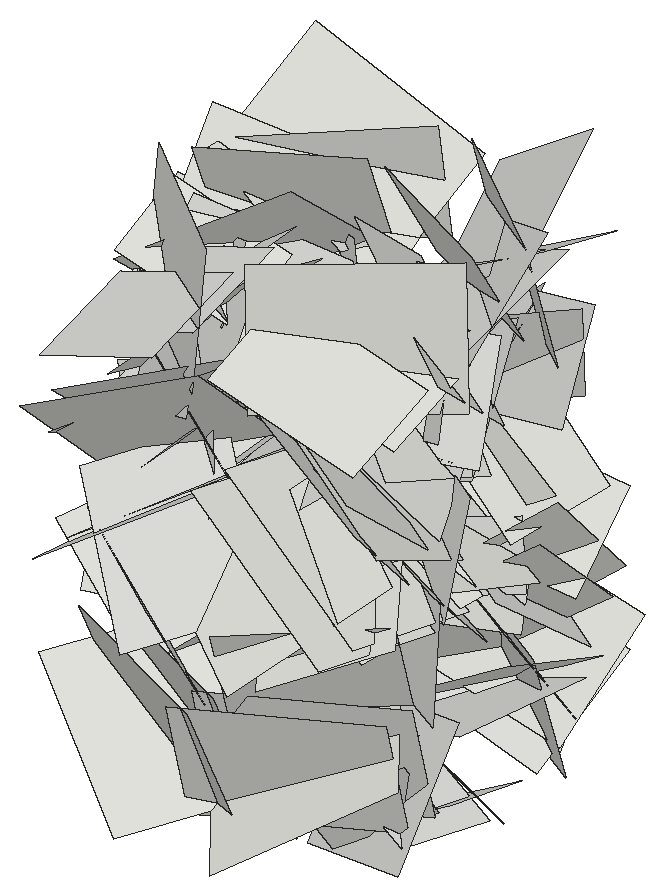
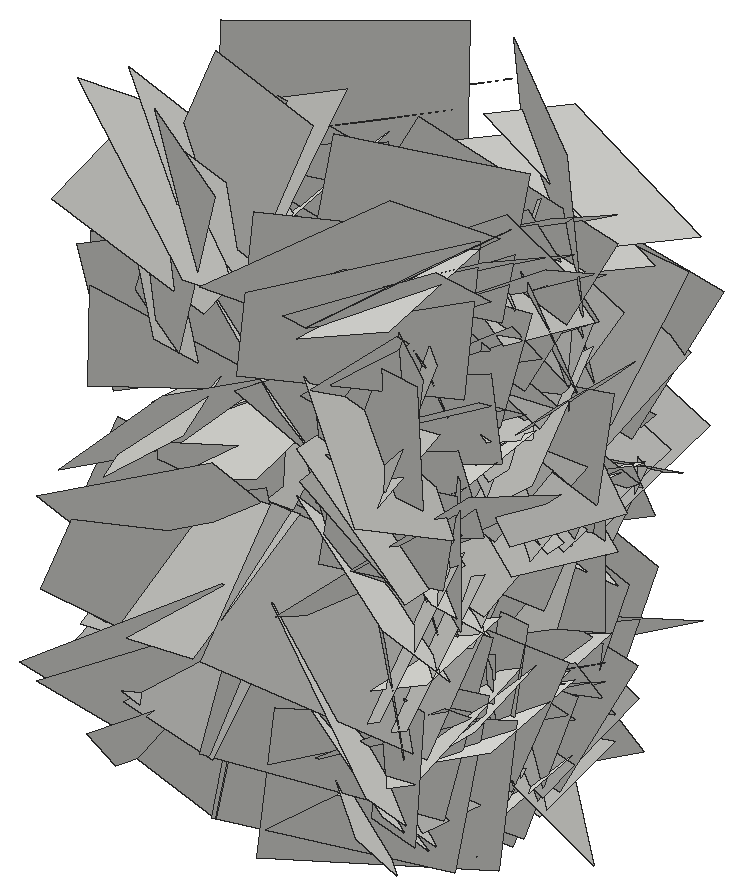
# SketchUp Ruby script. Lengths in inches.
U = 1.inch
M = Sketchup.active_model
def pt(a) = Geom::Point3d.new(a.map { |v| v * U })
def face(e, loops, mat)
  f = e.add_face(loops[0].map { |a| pt(a) })
  loops[1..].each { |l| e.add_face(l.map { |a| pt(a) }).erase! }
  f.material = f.back_material = mat if mat
  f
end
# faces: each face lists its corners as indices into pts; further lists are holes
def faces(e, pts, list, mat = nil) = list.each { |f| face(e, (f[0].is_a?(Array) ? f : [f]).map { |l| l.map { |i| pts[i] } }, mat) }
# xy, xz, yz: faces in a plane at the given z, y or x. An outline is a flat list of corners, or four numbers for a rectangle; further outlines are holes
def ring(l) = l.size == 4 ? [[l[0], l[1]], [l[2], l[1]], [l[2], l[3]], [l[0], l[3]]] : l.each_slice(2).to_a
def flat(e, list, mat, &to3) = list.each { |f| face(e, (f[0].is_a?(Array) ? f : [f]).map { |l| ring(l).map { |u, v| to3.(u, v) } }, mat) }
def xy(e, z, list, mat = nil) = flat(e, list, mat) { |x, y| [x, y, z] }
def xz(e, y, list, mat = nil) = flat(e, list, mat) { |x, z| [x, y, z] }
def yz(e, x, list, mat = nil) = flat(e, list, mat) { |y, z| [x, y, z] }
def lines(e, pts, list) = list.each { |a, b| e.add_line(pt(pts[a]), pt(pts[b])) }
# prism: a flat outline (further loops are holes) pulled along v
def prism(e, loops, v, mat = nil)
  f = face(e, loops, mat); d = Geom::Vector3d.new(v.map { |x| x * U })
  f.pushpull(f.normal.samedirection?(d) ? d.length : -d.length)
end
def box(e, o, s, mat = nil) = prism(e, [[o, [o[0] + s[0], o[1], o[2]], [o[0] + s[0], o[1] + s[1], o[2]], [o[0], o[1] + s[1], o[2]]]], [0, 0, s[2]], mat)
def at(x, y, z, deg = 0) = Geom::Transformation.translation(pt([x, y, z])) * Geom::Transformation.rotation(ORIGIN, Z_AXIS, deg.degrees)
def axes(o, x, y, z) = Geom::Transformation.new([*x, 0, *y, 0, *z, 0, *pt(o).to_a, 1])
def part(name) = M.definitions.add(name)
# library, detail: a bought-in or finely detailed component or shape, given as its bounding box
def library(name, o, s) = part(name).tap { |d| box(d.entities, o, s) }
def detail(e, o, s) = box(e.add_group.entities, o, s)
def put(e, d, t, mat = nil) = e.add_instance(d, t).tap { |i| i.material = mat if mat }
def group(e, t, mat = nil) = e.add_group.tap { |g| g.transformation = t; g.material = mat if mat }.entities
root = M.entities
c1 = part("Component\#6")
p = [[0.01,0,0],[0,3.24,4.54],[4.32,3.24,4.54],[4.33,0,0]]
faces(c1.entities,p,[[0,1,2,3]])
put(root,c1,axes([24.34,132.67,11.61],[-0.16439,-1.14375,-0.17253],[-0.24163,-0.14044,1.13591],[1.20204,-0.18465,0.20475]))
put(root,c1,axes([28.31,132.67,11.61],[0.16439,-1.14375,-0.17253],[0.24163,-0.14044,1.13591],[-1.20204,-0.18465,0.20475]))
put(root,c1,axes([24.34,126.24,11.02],[0.17433,0.41563,0.4957],[0.04437,0.50356,-0.43611],[0.68427,-0.13854,-0.09801]))
put(root,c1,axes([28.31,133.51,8.98],[0.15319,0.47062,-0.90401],[0.09722,-0.91536,-0.46187],[-1.07594,-0.0157,-0.17044]))
put(root,c1,axes([24.34,136.01,11.51],[0.06598,-0.27091,0.62957],[0.16839,0.62065,0.25136],[0.70672,-0.12259,-0.11867]))
put(root,c1,axes([24.34,130.2,1.79],[-0.1042,-0.77086,0.73803],[-0.17604,0.74317,0.75412],[1.11745,0.04519,0.18762]))
put(root,c1,axes([24.34,137.27,19.36],[-0.1763,0.15017,-0.9005],[0.15684,-0.89878,-0.17721],[0.95491,0.17535,-0.13715]))
put(root,c1,axes([28.31,136.42,13.64],[-0.14309,-0.55174,0.41683],[0.03038,0.41987,0.56505],[-0.73236,0.12522,-0.058]))
put(root,c1,axes([28.31,135.65,2.32],[0.1935,-1.06071,0.09437],[0.13048,0.11613,1.0671],[-1.12123,-0.16954,0.14047]))
put(root,c1,axes([24.34,132.96,18.89],[-0.10145,-0.91774,-0.17179],[0.02227,-0.17476,0.92192],[0.98945,-0.09016,-0.03837]))
put(root,c1,axes([24.34,133.07,14.74],[-0.12706,0.28525,0.91315],[0.02767,0.92092,-0.28425],[1.01369,0.01061,0.12222]))
put(root,c1,axes([24.34,135.14,15.06],[-0.15738,0.18416,-1.10832],[-0.16264,-1.1108,-0.16402],[1.17977,-0.12857,-0.17046]))
put(root,c1,axes([28.31,130.01,4.69],[-0.05447,0.12092,0.77662],[0.06993,0.77619,-0.11649],[-0.83019,0.05744,-0.06077]))
put(root,c1,axes([24.34,131.35,15.19],[0.02447,0.82058,-0.14823],[0.01236,-0.14859,-0.82075],[0.8838,-0.02064,0.01558]))
put(root,c1,axes([24.34,133.58,20.74],[-0.06025,0.71815,0.57437],[-0.00066,0.57544,-0.71955],[0.97476,0.04478,0.03501]))
put(root,c1,axes([24.34,133.14,16.06],[-0.03738,-0.31853,0.81486],[0.04959,0.81367,0.32009],[0.92608,-0.05642,0.01575]))
put(root,c1,axes([28.31,137.37,4.77],[0.01509,-0.67708,-0.46908],[0.05072,-0.46768,0.67651],[-0.87164,-0.03894,0.03124]))
put(root,c1,axes([24.34,128.53,16.93],[-0.30517,1.08519,-0.55956],[-0.1011,-0.59314,-1.10124],[1.29027,0.21019,-0.21864]))
put(root,c1,axes([24.34,127.92,4.7],[0.092,0.70183,0.2556],[0.07294,0.24871,-0.70628],[0.78837,-0.10491,0.03552]))
put(root,c1,axes([24.34,125.93,11.7],[0.16945,0.67455,-0.05214],[0.09647,-0.07453,-0.68517],[0.71064,-0.15073,0.10544]))
put(root,c1,axes([28.31,136.82,15.87],[0.16772,-0.74319,-0.48228],[-0.03783,-0.49486,0.75087],[-0.93836,-0.11289,-0.11647]))
put(root,c1,axes([28.31,131.86,3.01],[-0.01467,-0.55248,-0.51034],[0.00827,-0.51051,0.55244],[-0.7972,0.00487,0.01512]))
put(root,c1,axes([28.31,125.86,8.82],[-0.02658,0.53015,0.39509],[-0.11889,0.38623,-0.52538],[-0.69069,-0.08688,0.07523]))
put(root,c1,axes([24.34,127.95,5.4],[0.05879,0.74539,0.22064],[0.10629,0.21249,-0.74307],[0.81711,-0.08127,0.08079]))
put(root,c1,axes([28.31,131.99,-0.9375],[-0.0225,-0.54484,0.50649],[0.02225,0.50605,0.54525],[-0.78821,0.02984,0.00093]))
put(root,c1,axes([24.34,136.53,11.26],[-0.01536,-0.64622,-0.54667],[0.11065,-0.54394,0.64022],[0.89037,0.05645,-0.089]))
put(root,c1,axes([28.31,133.96,6.46],[0.0893,0.11056,0.97068],[0.19494,0.95507,-0.12474],[-1.01706,0.19277,0.06132]))
put(root,c1,axes([28.31,133.42,16.97],[0.14677,0.94615,0.46149],[0.22557,0.4307,-0.94687],[-1.09283,0.21597,-0.13346]))
put(root,c1,axes([24.34,127.34,21.1],[-0.03089,0.79811,0.32897],[0.11706,0.3299,-0.79059],[0.90753,-0.01539,0.11317]))
put(root,c1,axes([24.34,127.86,19.19],[-0.25173,1.01088,0.57921],[-0.04385,0.58343,-1.03521],[1.23418,0.22691,0.08136]))
put(root,c1,axes([28.31,129.8,15.91],[-0.05085,-0.71724,0.33006],[0.13843,0.31891,0.71198],[-0.82538,0.09767,0.09907]))
put(root,c1,axes([28.31,128.34,18.92],[-0.04874,0.38349,0.62334],[0.06251,0.62448,-0.37984],[-0.77325,0.02631,-0.07]))
put(root,c1,axes([24.34,132.55,10.48],[-0.11298,-1.07137,-0.22101],[-0.09706,-0.21254,1.07447],[1.1555,-0.12261,0.06864]))
put(root,c1,axes([28.31,129.18,10.77],[-0.08644,0.04023,-0.60323],[-0.06997,-0.60565,-0.03147],[-0.63702,0.06107,0.08531]))
put(root,c1,axes([24.34,132.5,3.06],[-0.12033,-0.77552,-0.96336],[-0.26418,-0.93322,0.78062],[1.28404,-0.26468,0.07033]))
put(root,c1,axes([28.31,129.23,5.41],[0.17398,-0.60139,0.60701],[-0.02487,0.6147,0.61536],[-0.9054,-0.13245,0.09973]))
put(root,c1,axes([28.31,130.03,2.94],[0.11679,-0.3481,0.76621],[0.04914,0.77408,0.34502],[-0.89071,-0.00294,0.1195]))
put(root,c1,axes([24.34,136.93,7.59],[-0.11136,0.24127,-0.97313],[0.07388,-0.97433,-0.24909],[1.06018,0.09324,-0.08486]))
put(root,c1,axes([28.31,133.88,6.93],[0.12434,-0.60409,0.41763],[-0.12699,0.40152,0.61444],[-0.76804,-0.16419,-0.03398]))
put(root,c1,axes([24.34,131.05,1.96],[-0.03915,-1.05631,0.36623],[-0.17317,0.36759,1.04378],[1.17236,0.01903,0.16641]))
put(root,c1,axes([24.34,133.1,9.3125],[-0.02086,0.87239,-0.16813],[0.14049,-0.16341,-0.8634],[0.93122,0.04419,0.12649]))
put(root,c1,axes([24.34,127.6,6.32],[0.09105,0.77875,-0.27248],[0.08108,-0.28029,-0.77696],[0.87078,-0.05533,0.10084]))
put(root,c1,axes([24.34,133.96,12.5],[0.03937,0.24323,0.81298],[0.12274,0.80469,-0.24604],[0.89109,-0.12158,-0.00203]))
put(root,c1,axes([28.31,132.63,6.14],[0.10731,0.87556,-0.00554],[0.12201,-0.01884,-0.87366],[-0.92006,0.09962,-0.1165]))
put(root,c1,axes([28.31,129.41,10.95],[0.18775,-0.48629,-0.69123],[-0.00245,-0.70652,0.49646],[-0.89586,-0.09998,-0.14623]))
put(root,c1,axes([24.34,129.45,15.69],[-0.00555,0.72683,0.86308],[-0.19522,0.85097,-0.71774],[1.18002,0.1442,-0.11468]))
put(root,c1,axes([28.31,129.84,16.13],[-0.05288,0.68465,0.04631],[0.09068,0.05228,-0.68068],[-0.72171,-0.04359,-0.08892]))
put(root,c1,axes([28.31,133.3125,17.59],[-0.01529,0.27468,0.5349],[-0.08187,0.52978,-0.27413],[-0.6321,-0.07526,0.02257]))
put(root,c1,axes([24.34,132.6,22.9],[0.05818,0.99288,0.05669],[-0.07779,0.06066,-0.99145],[1.05129,-0.05046,-0.07649]))
put(root,c1,axes([24.34,129.28,18.375],[0.15104,-0.37703,-0.77667],[-0.00911,-0.78776,0.38083],[0.9151,0.05438,0.13199]))
put(root,c1,axes([24.34,130.125,12.36],[-0.14413,1.23778,0.56401],[-0.30073,0.52855,-1.22835],[1.41013,0.23923,-0.20431]))
put(root,c1,axes([28.31,130.57,14.69],[0.08088,0.56373,-0.36339],[-0.06437,-0.35843,-0.56878],[-0.70803,0.09698,0.0102]))
put(root,c1,axes([28.31,131.53,3.64],[0.03356,0.34972,-0.55611],[-0.01458,-0.55628,-0.35061],[-0.69619,0.02851,-0.01946]))
put(root,c1,axes([24.34,133.79,15.82],[0.11741,-0.82822,-0.37202],[0.00882,-0.37384,0.83474],[0.96237,0.10447,0.03774]))
put(root,c1,axes([28.31,132.11,13.83],[0.12823,-0.67114,-0.46171],[0.10246,-0.45164,0.68184],[-0.85739,-0.15435,0.01243]))
put(root,c1,axes([24.34,128.52,17.74],[0.08604,0.43028,-0.81229],[0.04293,-0.81633,-0.42838],[0.97342,-0.00203,0.0907]))
put(root,c1,axes([28.31,134.57,7.51],[0.06425,-0.0713,-0.65597],[-0.02618,-0.65852,0.06929],[-0.69893,0.01811,-0.0629]))
put(root,c1,axes([24.34,133.2,0.29],[-0.16868,0.00753,1.30134],[-0.16064,1.302,-0.02607],[1.37005,0.15359,0.15716]))
put(root,c1,axes([28.31,127.28,0.51],[0.04452,-0.40985,0.5808],[0.07759,0.58122,0.40485],[-0.7495,0.03582,0.07641]))
put(root,c1,axes([24.34,129.68,16.21],[0.16446,-0.17941,-0.82447],[0.07006,-0.83314,0.19373],[0.89165,0.09856,0.13685]))
put(root,c1,axes([28.31,134.26,15.51],[0.13639,0.72841,-0.25059],[0.07067,-0.26364,-0.7321],[-0.81346,0.09922,-0.10562]))
put(root,c1,axes([24.34,128.87,2.92],[0.01411,0.95221,-0.19006],[0.11482,-0.19035,-0.94606],[1.02282,0.00823,0.10882]))
put(root,c1,axes([24.34,138.97,11.375],[-0.02639,-0.72989,-0.72722],[0.07911,-0.7268,0.72691],[1.08928,0.0351,-0.07041]))
put(root,c1,axes([24.34,131.74,20.5625],[-0.11289,-0.41624,-1.03402],[0.06809,-1.03929,0.41174],[1.17957,0.02016,-0.12272]))
put(root,c1,axes([28.31,131.9,7.66],[0.03371,0.19161,0.61883],[0.06203,0.6162,-0.1938],[-0.68388,0.06533,0.01292]))
put(root,c1,axes([24.34,134.95,12.42],[0.03363,0.92541,-1.00089],[-0.39451,-0.95725,-0.89685],[1.39004,-0.29406,-0.23032]))
put(root,c1,axes([28.31,131.8,8.64],[0.08497,0.05507,0.67491],[0.04101,0.67814,-0.05993],[-0.71661,0.04534,0.0766]))
put(root,c1,axes([24.34,137.87,11.82],[0.23548,-0.98581,-0.19043],[-0.17104,-0.22756,0.98976],[1.05044,0.18394,0.20385]))
put(root,c1,axes([24.34,129.625,19.87],[-0.14331,0.9196,0.97349],[-0.15794,0.96203,-0.92947],[1.41069,0.20113,-0.00516]))
put(root,c1,axes([24.34,130.99,8.6],[0.04494,-0.64922,0.68663],[0.20873,0.6783,0.62918],[0.97967,-0.11474,-0.16555]))
put(root,c1,axes([24.34,133.91,11.1875],[-0.02059,0.92356,-0.8814],[-0.20413,-0.87353,-0.91107],[1.33776,-0.11908,-0.15259]))
put(root,c1,axes([24.34,128.56,10.3125],[-0.23413,0.04823,1.24691],[0.1221,1.26168,-0.02839],[1.31707,-0.10839,0.22429]))
put(root,c1,axes([24.34,131.94,16.85],[-0.08825,-0.96476,0.81898],[-0.08011,0.82307,0.9619],[1.33903,-0.01434,0.11152]))
put(root,c1,axes([24.34,131.18,15.16],[0.15294,-1.16278,0.39158],[-0.28955,0.35393,1.15166],[1.26792,0.22109,0.21577]))
put(root,c1,axes([28.31,134.77,2.57],[0.05447,0.40704,0.46107],[0.08155,0.45478,-0.41007],[-0.64681,0.09162,-0.01288]))
put(root,c1,axes([24.34,134.14,22.88],[0.03825,0.99518,-0.25742],[0.13842,-0.25993,-0.98657],[1.08078,-0.00193,0.13547]))
put(root,c1,axes([23.62,124.93,11.12],[0.54058,0.75668,0.32998],[0.30141,0.20311,-0.90522],[0.82148,-0.57246,0.11499]))
put(root,c1,axes([24.34,127.92,6.47],[-0.03611,0.05394,1.13531],[0.09971,1.13206,-0.05096],[1.20066,-0.09239,0.03838]))
put(root,c1,axes([28.31,138.1,17.99],[0.00934,-0.49027,-0.41508],[0.1892,-0.3969,0.47259],[-0.65411,-0.1218,0.13076]))
put(root,c1,axes([24.34,127.69,20.12],[-0.02742,-1.01137,-0.35231],[0.21232,-0.35076,0.99222],[1.1152,0.04191,-0.19757]))
put(root,c1,axes([24.34,130,20.12],[-0.02742,-1.01137,-0.35231],[0.21232,-0.35076,0.99222],[1.1152,0.04191,-0.19757]))
put(root,c1,axes([28.31,129.35,18.22],[0.07955,-0.40219,0.442],[0.06566,0.44831,0.39741],[-0.63004,-0.00406,0.09723]))
put(root,c1,axes([24.34,129.81,24.32],[-0.08615,-0.07511,-1.33483],[-0.12267,-1.33188,0.08199],[1.41184,-0.12031,-0.07433]))
put(root,c1,axes([24.34,131.16,1.32],[0.11103,-1.00768,0.14491],[0.13016,0.15712,1.00381],[1.07125,0.08535,-0.13699]))
put(root,c1,axes([24.34,136.29,19.65],[0.239,0.33681,-1.04778],[-0.13934,-1.05364,-0.36698],[1.15826,-0.19625,0.17205]))
put(root,c1,axes([24.34,129.42,5.47],[-0.26825,1.30607,0.06413],[0.25565,0.11082,-1.30519],[1.36232,0.23638,0.25756]))
put(root,c1,axes([24.34,126.61,12.8],[-0.1414,-0.87971,0.87765],[0.19082,0.8597,0.88908],[1.30331,-0.22132,-0.03495]))
put(root,c1,axes([24.34,133.96,9.66],[0.06967,-1.04066,0.34132],[0.1454,0.34706,1.03175],[1.15177,0.01914,-0.15089]))
put(root,c1,axes([24.34,134.94,17.85],[0.08672,-0.29938,1.1859],[-0.04442,1.18717,0.30259],[1.29573,0.06074,-0.069]))
put(root,c1,axes([24.34,129.48,20.64],[-0.14207,1.22324,0.51937],[0.11373,0.53026,-1.2212],[1.40407,0.08082,0.15147]))
put(root,c1,axes([24.34,129.66,12.47],[-0.1081,-1.2535,0.58167],[-0.00417,0.58351,1.25678],[1.46479,-0.09085,0.0465]))
put(root,c1,axes([24.34,125.82,11.42],[0.20547,0.4933,-0.99975],[0.03886,-1.01702,-0.49472],[1.18108,-0.05236,0.1902]))
put(root,c1,axes([24.34,131.95,0.87],[0.07095,-0.70744,0.83659],[0.30432,0.82019,0.6706],[1.12076,-0.17792,-0.23504]))
put(root,c1,axes([24.34,139.8125,5.82],[0.12038,-0.94885,-0.86303],[-0.08352,-0.86993,0.94607],[1.35702,0.03063,0.13479]))
put(root,c1,axes([24.34,133.04,19.75],[0.14526,-0.49923,0.95494],[0.24012,0.95446,0.46647],[1.11669,-0.1403,-0.22453]))
put(root,c1,axes([24.34,128.24,17.68],[0.22785,0.52614,1.07761],[-0.06777,1.09826,-0.52347],[1.26934,-0.03581,-0.22138]))
put(root,c1,axes([24.34,133.15,22.79],[0.15509,1.06813,0.73269],[-0.10614,0.74447,-1.06531],[1.36888,-0.06329,-0.16562]))
put(root,c1,axes([24.34,132.12,7.08],[-0.00585,1.22451,-0.43101],[0.11167,-0.42917,-1.22063],[1.3715,0.04016,0.09755]))
put(root,c1,axes([24.34,125.99,1.35],[0.00241,0.79041,1.08039],[0.06651,1.07914,-0.78963],[1.41741,-0.05198,0.03522]))
put(root,c1,axes([24.34,127.67,13.74],[0.06329,-0.97705,0.81505],[0.12838,0.8166,0.97005],[1.34259,-0.03203,-0.13118]))
put(root,c1,axes([24.34,137,19.49],[0.23927,-0.1296,-1.18474],[0.04055,-1.20439,0.13904],[1.26266,0.06324,0.22004]))
put(root,c1,axes([24.34,135.39,1.18],[0.01455,-0.40823,1.27358],[0.1801,1.26386,0.40328],[1.40617,-0.15765,-0.06483]))
put(root,c1,axes([24.34,128.0625,10.23],[0.10909,-1.3698,0.20566],[-0.00727,0.20572,1.37363],[1.46824,0.1028,-0.00848]))
put(root,c1,axes([24.34,129.98,10.23],[0.10909,-1.3698,0.20566],[-0.00727,0.20572,1.37363],[1.46824,0.1028,-0.00848]))
put(root,c1,axes([24.34,138.98,4.78],[0.22268,-0.9196,-0.8307],[0.07298,-0.83259,0.9391],[1.31157,0.20246,0.08879]))
put(root,c1,axes([23.17,124.5,5.79],[0.83668,1.07369,0.2523],[0.21003,0.16716,-1.33127],[1.15009,-0.81162,0.05958]))
put(root,c1,axes([24.34,130.78,10.54],[0.24762,-1.26357,-0.1726],[-0.00687,-0.17664,1.28442],[1.3518,0.23056,0.03815]))
put(root,c1,axes([24.34,136.82,5.83],[0.1656,-1.02965,0.80161],[0.14776,0.81588,1.02082],[1.37528,0.03632,-0.2062]))
put(root,c1,axes([24.34,130.15,15.41],[0.24379,0.89731,1.03665],[0.02149,1.04879,-0.91232],[1.45316,-0.16605,-0.16042]))
put(root,c1,axes([24.34,135.96,3.29],[0.1622,-0.76384,1.11136],[0.23079,1.11781,0.7383],[1.4107,-0.09505,-0.24857]))
put(root,c1,axes([24.34,125.3125,7.6875],[0.15543,0.49215,-1.26812],[0.29157,-1.25984,-0.45713],[1.41209,0.20597,0.23397]))
put(root,c1,axes([24.34,126.76,7.6875],[0.15543,0.49215,-1.26812],[0.29157,-1.25984,-0.45713],[1.41209,0.20597,0.23397]))
put(root,c1,axes([24.23,125.5,13.2],[1.07209,0.56535,0.5401],[0.40295,0.41611,-1.14744],[0.72423,-1.06841,-0.1611]))
put(root,c1,axes([38.22,125.5,13.2],[-1.07209,0.56535,0.5401],[-0.40295,0.41611,-1.14744],[-0.72423,-1.06841,-0.1611]))
put(root,c1,axes([38.11,126.76,7.6875],[-0.15543,0.49215,-1.26812],[-0.29157,-1.25984,-0.45713],[-1.41209,0.20597,0.23397]))
put(root,c1,axes([38.11,125.3125,7.6875],[-0.15543,0.49215,-1.26812],[-0.29157,-1.25984,-0.45713],[-1.41209,0.20597,0.23397]))
put(root,c1,axes([38.11,135.96,3.29],[-0.1622,-0.76384,1.11136],[-0.23079,1.11781,0.7383],[-1.4107,-0.09505,-0.24857]))
put(root,c1,axes([38.11,130.15,15.41],[-0.24379,0.89731,1.03665],[-0.02149,1.04879,-0.91232],[-1.45316,-0.16605,-0.16042]))
put(root,c1,axes([38.11,136.82,5.83],[-0.1656,-1.02965,0.80161],[-0.14776,0.81588,1.02082],[-1.37528,0.03632,-0.2062]))
put(root,c1,axes([38.11,130.78,10.54],[-0.24762,-1.26357,-0.1726],[0.00687,-0.17664,1.28442],[-1.3518,0.23056,0.03815]))
put(root,c1,axes([39.28,124.5,5.79],[-0.83668,1.07369,0.2523],[-0.21003,0.16716,-1.33127],[-1.15009,-0.81162,0.05958]))
put(root,c1,axes([38.11,138.98,4.78],[-0.22268,-0.9196,-0.8307],[-0.07298,-0.83259,0.9391],[-1.31157,0.20246,0.08879]))
put(root,c1,axes([38.11,128.0625,10.23],[-0.10909,-1.3698,0.20566],[0.00727,0.20572,1.37363],[-1.46824,0.1028,-0.00848]))
put(root,c1,axes([38.11,129.98,10.23],[-0.10909,-1.3698,0.20566],[0.00727,0.20572,1.37363],[-1.46824,0.1028,-0.00848]))
put(root,c1,axes([38.11,135.39,1.18],[-0.01455,-0.40823,1.27358],[-0.1801,1.26386,0.40328],[-1.40617,-0.15765,-0.06483]))
put(root,c1,axes([38.11,137,19.49],[-0.23927,-0.1296,-1.18474],[-0.04055,-1.20439,0.13904],[-1.26266,0.06324,0.22004]))
put(root,c1,axes([38.11,127.67,13.74],[-0.06329,-0.97705,0.81505],[-0.12838,0.8166,0.97005],[-1.34259,-0.03203,-0.13118]))
put(root,c1,axes([38.11,125.99,1.35],[-0.00241,0.79041,1.08039],[-0.06651,1.07914,-0.78963],[-1.41741,-0.05198,0.03522]))
put(root,c1,axes([38.11,132.12,7.08],[0.00585,1.22451,-0.43101],[-0.11167,-0.42917,-1.22063],[-1.3715,0.04016,0.09755]))
put(root,c1,axes([38.11,133.15,22.79],[-0.15509,1.06813,0.73269],[0.10614,0.74447,-1.06531],[-1.36888,-0.06329,-0.16562]))
put(root,c1,axes([38.11,128.24,17.68],[-0.22785,0.52614,1.07761],[0.06777,1.09826,-0.52347],[-1.26934,-0.03581,-0.22138]))
put(root,c1,axes([38.11,133.04,19.75],[-0.14526,-0.49923,0.95494],[-0.24012,0.95446,0.46647],[-1.11669,-0.1403,-0.22453]))
put(root,c1,axes([38.11,139.8125,5.82],[-0.12038,-0.94885,-0.86303],[0.08352,-0.86993,0.94607],[-1.35702,0.03063,0.13479]))
put(root,c1,axes([38.11,131.95,0.87],[-0.07095,-0.70744,0.83659],[-0.30432,0.82019,0.6706],[-1.12076,-0.17792,-0.23504]))
put(root,c1,axes([38.11,125.82,11.42],[-0.20547,0.4933,-0.99975],[-0.03886,-1.01702,-0.49472],[-1.18108,-0.05236,0.1902]))
put(root,c1,axes([38.11,129.66,12.47],[0.1081,-1.2535,0.58167],[0.00417,0.58351,1.25678],[-1.46479,-0.09085,0.0465]))
put(root,c1,axes([38.11,129.48,20.64],[0.14207,1.22324,0.51937],[-0.11373,0.53026,-1.2212],[-1.40407,0.08082,0.15147]))
put(root,c1,axes([38.11,134.94,17.85],[-0.08672,-0.29938,1.1859],[0.04442,1.18717,0.30259],[-1.29573,0.06074,-0.069]))
put(root,c1,axes([38.11,133.96,9.66],[-0.06967,-1.04066,0.34132],[-0.1454,0.34706,1.03175],[-1.15177,0.01914,-0.15089]))
put(root,c1,axes([38.11,126.61,12.8],[0.1414,-0.87971,0.87765],[-0.19082,0.8597,0.88908],[-1.30331,-0.22132,-0.03495]))
put(root,c1,axes([38.11,129.42,5.47],[0.26825,1.30607,0.06413],[-0.25565,0.11082,-1.30519],[-1.36232,0.23638,0.25756]))
put(root,c1,axes([38.11,136.29,19.65],[-0.239,0.33681,-1.04778],[0.13934,-1.05364,-0.36698],[-1.15826,-0.19625,0.17205]))
put(root,c1,axes([38.11,131.16,1.32],[-0.11103,-1.00768,0.14491],[-0.13016,0.15712,1.00381],[-1.07125,0.08535,-0.13699]))
put(root,c1,axes([38.11,129.81,24.32],[0.08615,-0.07511,-1.33483],[0.12267,-1.33188,0.08199],[-1.41184,-0.12031,-0.07433]))
put(root,c1,axes([34.14,129.35,18.22],[-0.07955,-0.40219,0.442],[-0.06566,0.44831,0.39741],[0.63004,-0.00406,0.09723]))
put(root,c1,axes([38.11,127.69,20.12],[0.02742,-1.01137,-0.35231],[-0.21232,-0.35076,0.99222],[-1.1152,0.04191,-0.19757]))
put(root,c1,axes([38.11,130,20.12],[0.02742,-1.01137,-0.35231],[-0.21232,-0.35076,0.99222],[-1.1152,0.04191,-0.19757]))
put(root,c1,axes([34.14,138.1,17.99],[-0.00934,-0.49027,-0.41508],[-0.1892,-0.3969,0.47259],[0.65411,-0.1218,0.13076]))
put(root,c1,axes([38.11,127.92,6.47],[0.03611,0.05394,1.13531],[-0.09971,1.13206,-0.05096],[-1.20066,-0.09239,0.03838]))
put(root,c1,axes([38.83,124.93,11.12],[-0.54058,0.75668,0.32998],[-0.30141,0.20311,-0.90522],[-0.82148,-0.57246,0.11499]))
put(root,c1,axes([38.11,134.14,22.88],[-0.03825,0.99518,-0.25742],[-0.13842,-0.25993,-0.98657],[-1.08078,-0.00193,0.13547]))
put(root,c1,axes([34.14,134.77,2.57],[-0.05447,0.40704,0.46107],[-0.08155,0.45478,-0.41007],[0.64681,0.09162,-0.01288]))
put(root,c1,axes([38.11,131.18,15.16],[-0.15294,-1.16278,0.39158],[0.28955,0.35393,1.15166],[-1.26792,0.22109,0.21577]))
put(root,c1,axes([38.11,131.94,16.85],[0.08825,-0.96476,0.81898],[0.08011,0.82307,0.9619],[-1.33903,-0.01434,0.11152]))
put(root,c1,axes([38.11,128.56,10.3125],[0.23413,0.04823,1.24691],[-0.1221,1.26168,-0.02839],[-1.31707,-0.10839,0.22429]))
put(root,c1,axes([38.11,133.91,11.1875],[0.02059,0.92356,-0.8814],[0.20413,-0.87353,-0.91107],[-1.33776,-0.11908,-0.15259]))
put(root,c1,axes([38.11,130.99,8.6],[-0.04494,-0.64922,0.68663],[-0.20873,0.6783,0.62918],[-0.97967,-0.11474,-0.16555]))
put(root,c1,axes([38.11,129.625,19.87],[0.14331,0.9196,0.97349],[0.15794,0.96203,-0.92947],[-1.41069,0.20113,-0.00516]))
put(root,c1,axes([38.11,137.87,11.82],[-0.23548,-0.98581,-0.19043],[0.17104,-0.22756,0.98976],[-1.05044,0.18394,0.20385]))
put(root,c1,axes([34.14,131.8,8.64],[-0.08497,0.05507,0.67491],[-0.04101,0.67814,-0.05993],[0.71661,0.04534,0.0766]))
put(root,c1,axes([38.11,134.95,12.42],[-0.03363,0.92541,-1.00089],[0.39451,-0.95725,-0.89685],[-1.39004,-0.29406,-0.23032]))
put(root,c1,axes([34.14,131.9,7.66],[-0.03371,0.19161,0.61883],[-0.06203,0.6162,-0.1938],[0.68388,0.06533,0.01292]))
put(root,c1,axes([38.11,131.74,20.5625],[0.11289,-0.41624,-1.03402],[-0.06809,-1.03929,0.41174],[-1.17957,0.02016,-0.12272]))
put(root,c1,axes([38.11,138.97,11.375],[0.02639,-0.72989,-0.72722],[-0.07911,-0.7268,0.72691],[-1.08928,0.0351,-0.07041]))
put(root,c1,axes([38.11,128.87,2.92],[-0.01411,0.95221,-0.19006],[-0.11482,-0.19035,-0.94606],[-1.02282,0.00823,0.10882]))
put(root,c1,axes([34.14,134.26,15.51],[-0.13639,0.72841,-0.25059],[-0.07067,-0.26364,-0.7321],[0.81346,0.09922,-0.10562]))
put(root,c1,axes([38.11,129.68,16.21],[-0.16446,-0.17941,-0.82447],[-0.07006,-0.83314,0.19373],[-0.89165,0.09856,0.13685]))
put(root,c1,axes([34.14,127.28,0.51],[-0.04452,-0.40985,0.5808],[-0.07759,0.58122,0.40485],[0.7495,0.03582,0.07641]))
